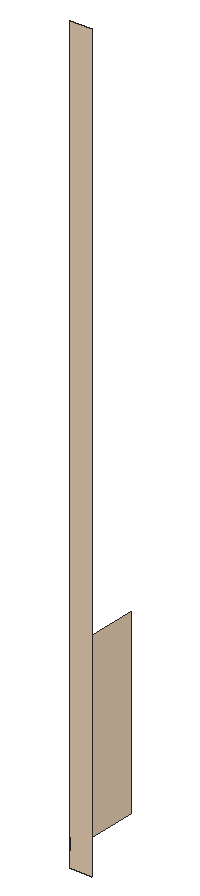
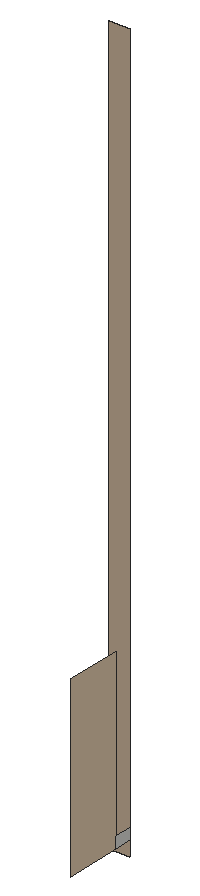
# SketchUp Ruby script. Lengths in inches.
U = 1.inch
M = Sketchup.active_model
def pt(a) = Geom::Point3d.new(a.map { |v| v * U })
def face(e, loops, mat)
  f = e.add_face(loops[0].map { |a| pt(a) })
  loops[1..].each { |l| e.add_face(l.map { |a| pt(a) }).erase! }
  f.material = f.back_material = mat if mat
  f
end
# faces: each face lists its corners as indices into pts; further lists are holes
def faces(e, pts, list, mat = nil) = list.each { |f| face(e, (f[0].is_a?(Array) ? f : [f]).map { |l| l.map { |i| pts[i] } }, mat) }
# xy, xz, yz: faces in a plane at the given z, y or x. An outline is a flat list of corners, or four numbers for a rectangle; further outlines are holes
def ring(l) = l.size == 4 ? [[l[0], l[1]], [l[2], l[1]], [l[2], l[3]], [l[0], l[3]]] : l.each_slice(2).to_a
def flat(e, list, mat, &to3) = list.each { |f| face(e, (f[0].is_a?(Array) ? f : [f]).map { |l| ring(l).map { |u, v| to3.(u, v) } }, mat) }
def xy(e, z, list, mat = nil) = flat(e, list, mat) { |x, y| [x, y, z] }
def xz(e, y, list, mat = nil) = flat(e, list, mat) { |x, z| [x, y, z] }
def yz(e, x, list, mat = nil) = flat(e, list, mat) { |y, z| [x, y, z] }
def lines(e, pts, list) = list.each { |a, b| e.add_line(pt(pts[a]), pt(pts[b])) }
# prism: a flat outline (further loops are holes) pulled along v
def prism(e, loops, v, mat = nil)
  f = face(e, loops, mat); d = Geom::Vector3d.new(v.map { |x| x * U })
  f.pushpull(f.normal.samedirection?(d) ? d.length : -d.length)
end
def box(e, o, s, mat = nil) = prism(e, [[o, [o[0] + s[0], o[1], o[2]], [o[0] + s[0], o[1] + s[1], o[2]], [o[0], o[1] + s[1], o[2]]]], [0, 0, s[2]], mat)
def at(x, y, z, deg = 0) = Geom::Transformation.translation(pt([x, y, z])) * Geom::Transformation.rotation(ORIGIN, Z_AXIS, deg.degrees)
def axes(o, x, y, z) = Geom::Transformation.new([*x, 0, *y, 0, *z, 0, *pt(o).to_a, 1])
def part(name) = M.definitions.add(name)
# library, detail: a bought-in or finely detailed component or shape, given as its bounding box
def library(name, o, s) = part(name).tap { |d| box(d.entities, o, s) }
def detail(e, o, s) = box(e.add_group.entities, o, s)
def put(e, d, t, mat = nil) = e.add_instance(d, t).tap { |i| i.material = mat if mat }
def group(e, t, mat = nil) = e.add_group.tap { |g| g.transformation = t; g.material = mat if mat }.entities
root = M.entities
M.materials.add("[0012_Bisque]").color = [234, 209, 180]
M.materials.add("[0012_Bisque]1").color = [237, 212, 182]
xz(root,364.57,[[376.86,95.625,388.14,490.375]],"[0012_Bisque]")
yz(root,376.86,[[364.57,103.6875,374.19,109.8125]])
yz(root,376.86,[[374.19,103.6875,403.76,197.75]],"[0012_Bisque]1")
